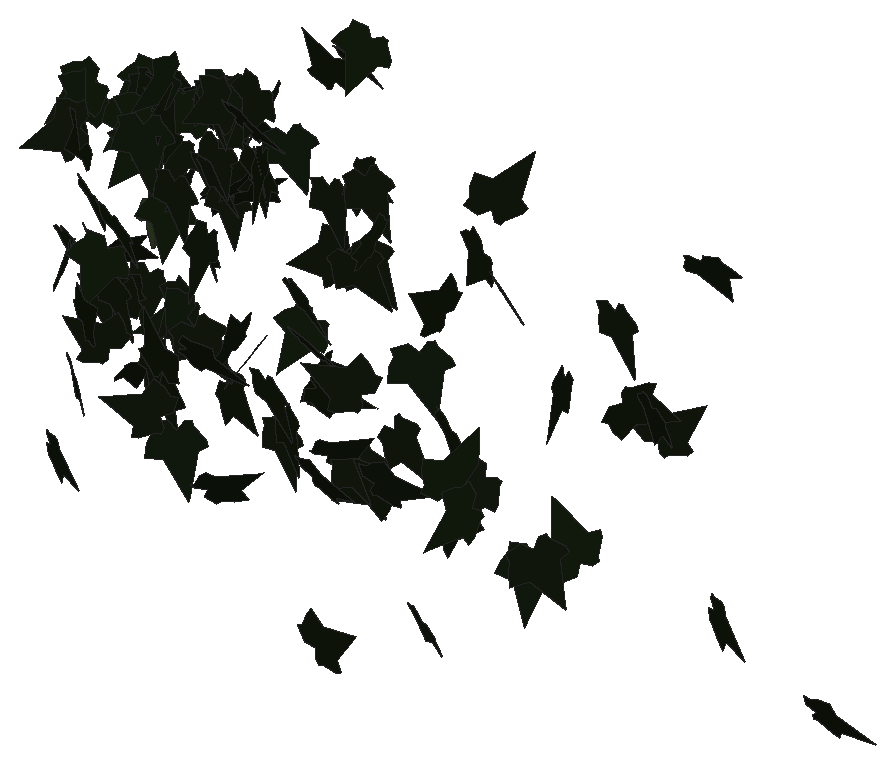
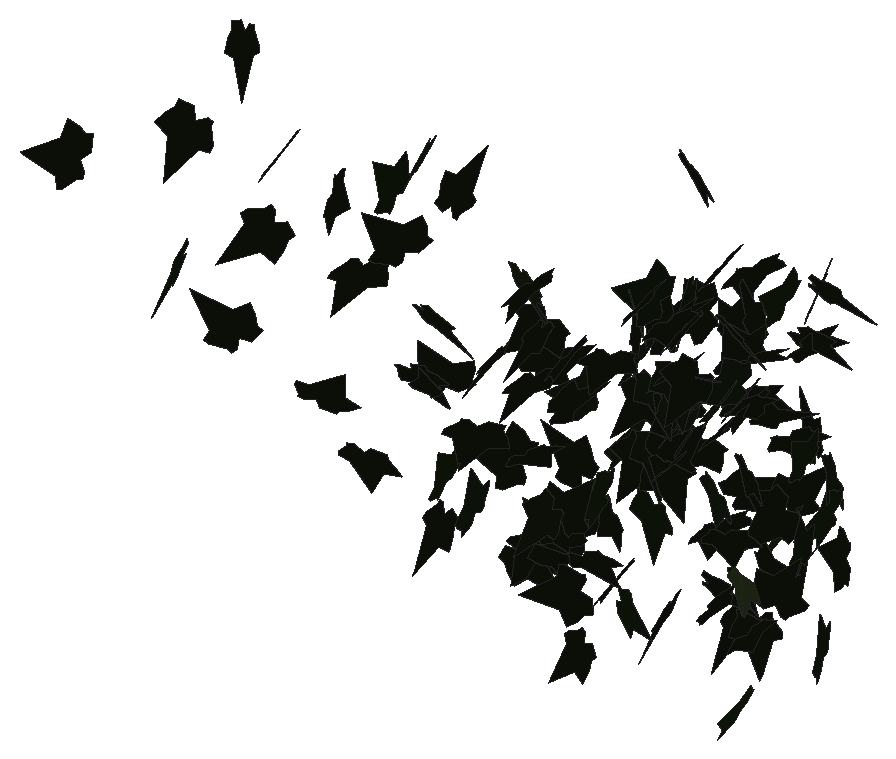
# SketchUp Ruby script. Lengths in inches.
U = 1.inch
M = Sketchup.active_model
def pt(a) = Geom::Point3d.new(a.map { |v| v * U })
def face(e, loops, mat)
  f = e.add_face(loops[0].map { |a| pt(a) })
  loops[1..].each { |l| e.add_face(l.map { |a| pt(a) }).erase! }
  f.material = f.back_material = mat if mat
  f
end
# faces: each face lists its corners as indices into pts; further lists are holes
def faces(e, pts, list, mat = nil) = list.each { |f| face(e, (f[0].is_a?(Array) ? f : [f]).map { |l| l.map { |i| pts[i] } }, mat) }
# xy, xz, yz: faces in a plane at the given z, y or x. An outline is a flat list of corners, or four numbers for a rectangle; further outlines are holes
def ring(l) = l.size == 4 ? [[l[0], l[1]], [l[2], l[1]], [l[2], l[3]], [l[0], l[3]]] : l.each_slice(2).to_a
def flat(e, list, mat, &to3) = list.each { |f| face(e, (f[0].is_a?(Array) ? f : [f]).map { |l| ring(l).map { |u, v| to3.(u, v) } }, mat) }
def xy(e, z, list, mat = nil) = flat(e, list, mat) { |x, y| [x, y, z] }
def xz(e, y, list, mat = nil) = flat(e, list, mat) { |x, z| [x, y, z] }
def yz(e, x, list, mat = nil) = flat(e, list, mat) { |y, z| [x, y, z] }
def lines(e, pts, list) = list.each { |a, b| e.add_line(pt(pts[a]), pt(pts[b])) }
# prism: a flat outline (further loops are holes) pulled along v
def prism(e, loops, v, mat = nil)
  f = face(e, loops, mat); d = Geom::Vector3d.new(v.map { |x| x * U })
  f.pushpull(f.normal.samedirection?(d) ? d.length : -d.length)
end
def box(e, o, s, mat = nil) = prism(e, [[o, [o[0] + s[0], o[1], o[2]], [o[0] + s[0], o[1] + s[1], o[2]], [o[0], o[1] + s[1], o[2]]]], [0, 0, s[2]], mat)
def at(x, y, z, deg = 0) = Geom::Transformation.translation(pt([x, y, z])) * Geom::Transformation.rotation(ORIGIN, Z_AXIS, deg.degrees)
def axes(o, x, y, z) = Geom::Transformation.new([*x, 0, *y, 0, *z, 0, *pt(o).to_a, 1])
def part(name) = M.definitions.add(name)
# library, detail: a bought-in or finely detailed component or shape, given as its bounding box
def library(name, o, s) = part(name).tap { |d| box(d.entities, o, s) }
def detail(e, o, s) = box(e.add_group.entities, o, s)
def put(e, d, t, mat = nil) = e.add_instance(d, t).tap { |i| i.material = mat if mat }
def group(e, t, mat = nil) = e.add_group.tap { |g| g.transformation = t; g.material = mat if mat }.entities
root = M.entities
M.materials.add("efeu1").color = [18, 25, 13]
M.materials.add("efeu2").color = [43, 57, 29]
c1 = part("ivyleaf_9")
p = [[1.54,2.16,1.25],[1.36,2.04,1.19],[-0.21,0.99,0.68],[-0.71,1.11,0.82],[-0.85,0.86,0.67],[-0.8,0.17,0.21],
  [-0.9,-0.01,0.1],[-0.67,-0.16,-0.02],[-0.08,-0.08,-0.05],[-0.03,-0.6,-0.4],[0.65,-0.88,-0.66],[0.83,-0.6,-0.49],
  [1.29,-0.42,-0.43],[1.8125,-0.07,-0.26],[1.21,0.44,0.15]]
faces(c1.entities,p,[[0,1,2,3,4,5,6,7,8,9,10,11,12,13,14]],"efeu1")
c2 = part("ivyleaf_10")
p = [[0,0.5,-0.03],[-0.0625,2.02,-0.43],[-0.19,2.01,-0.46],[-0.54,1.05,-0.29],[-0.52,0.625,-0.18],[-0.83,0.76,-0.28],
  [-1.16,0.64,-0.33],[-1.15,0.33,-0.24],[-0.77,-0.39,0.02],[-0.3,-0.51,0.16],[0.04,-0.48,0.23],[-0.02,2.01,-0.4375],
  [-0.06,2.01,-0.43],[0.04,-0.49,0.23],[0.67,-0.49,0.14],[1.38,0.36,-0.2],[1.375,0.51,-0.24],[0.81,0.65,-0.19],
  [0.62,0.59,-0.15],[0.6,1.09,-0.28],[0.5,1.23,-0.31]]
faces(c2.entities,p,[[0,1,2,3,4,5,6,7,8,9,10],[11,12,0,13,14,15,16,17,18,19,20]],"efeu2")
put(root,c1,axes([640.31,116.39,317.35],[1.16846,-0.88159,0.07129],[0.0667,-0.02996,-1.46364],[0.88195,1.17025,0.01624]))
put(root,c2,axes([640.9,124.67,315.8],[1.22207,-0.2873,0.16471],[0.19934,0.13529,-1.24301],[0.26445,1.22568,0.17581]))
put(root,c1,axes([641.4,136.23,319.18],[-0.91834,0.42729,-0.85127],[0.67528,-0.54188,-1.00047],[-0.67174,-1.12888,0.15803]))
put(root,c1,axes([640.67,119,315.09],[-0.02679,-0.37717,1.31538],[0.43757,-1.24892,-0.3492],[1.29654,0.41371,0.14503]))
put(root,c1,axes([641.8,120.08,312.01],[0.79627,-0.16263,1.10794],[-1.07914,0.25165,0.8125],[-0.29908,-1.34099,0.01811]))
put(root,c1,axes([641.22,123.75,311.48],[-0.09051,-1.27467,0.05842],[-0.03626,-0.05597,-1.27747],[1.27549,-0.09204,-0.03217]))
put(root,c1,axes([640.7,116.8125,307.07],[0.74096,-0.60878,-1.0482],[1.0596,-0.27136,0.90663],[-0.58871,-1.25464,0.31252]))
put(root,c1,axes([641.52,123.4375,323.16],[-0.67849,-0.09135,-1.09196],[1.09327,0.03031,-0.68184],[0.07401,-1.28522,0.06154]))
put(root,c1,axes([643.01,120.47,325.32],[-0.81227,0.08622,1.0327],[-1.00974,-0.36095,-0.76408],[0.23307,-1.26331,0.28879]))
put(root,c1,axes([642.73,116.17,329.4],[-1.35533,-0.27286,0.18589],[-0.17869,-0.05418,-1.38241],[0.27763,-1.36694,0.01768]))
put(root,c1,axes([641.59,117.83,313.6875],[0.61437,-1.24201,-0.09434],[-0.03171,0.08956,-1.3856],[1.24518,0.61508,0.01126]))
put(root,c1,axes([642.71,116.11,328.61],[-0.69237,-0.92516,0.77717],[-0.40045,-0.6694,-1.15362],[1.13998,-0.79705,0.06677]))
put(root,c1,axes([643.08,112.52,317.27],[-0.08249,0.66584,1.14036],[-0.08995,1.13709,-0.67044],[-1.31745,-0.11932,-0.02563]))
put(root,c1,axes([642.71,122.59,327.22],[-0.73308,-1.09231,0.05257],[0.08551,-0.12035,-1.30825],[1.09023,-0.72504,0.13796]))
put(root,c1,axes([642.05,116.9,320.68],[0.35585,-0.86092,0.90075],[0.43721,-0.79093,-0.92868],[1.16678,0.55894,0.07327]))
put(root,c1,axes([644.05,118.01,312.32],[-0.11258,0.1104,1.3975],[-0.92093,1.05121,-0.15723],[-1.05692,-0.92771,-0.01186]))
put(root,c1,axes([642.74,121.86,326.74],[0.37173,-1.3592,-0.17061],[-0.02655,0.1696,-1.40899],[1.36961,0.37219,0.01899]))
put(root,c1,axes([643.38,123.22,317.7],[-0.80166,-0.87771,-0.50482],[0.34134,0.37192,-1.18872],[0.95326,-0.87131,0.00112]))
put(root,c1,axes([642.87,122.73,304.78],[0.64586,-1.21892,0.28644],[0.15296,-0.24308,-1.3793],[1.24274,0.6634,0.02091]))
put(root,c1,axes([643.11,121.95,327.26],[0.44784,-1.22621,0.06593],[0.02248,-0.06198,-1.30544],[1.22778,0.44841,-0.00014]))
put(root,c1,axes([644.16,120.07,326.11],[-0.9206,-0.80956,0.49178],[-0.3784,-0.31436,-1.22586],[0.86836,-0.99526,-0.01283]))
put(root,c1,axes([643.47,117.37,316.88],[0.79356,0.92156,0.60672],[0.39451,0.46094,-1.21614],[-1.03041,0.88621,0.00163]))
put(root,c1,axes([644.75,118.34,308.8125],[0.09794,1.27164,-0.20626],[-0.02176,-0.20519,-1.27539],[-1.28807,0.10015,0.00587]))
put(root,c1,axes([643.85,116.56,315.11],[0.72763,-1.21166,0.00874],[0.00123,-0.00945,-1.41335],[1.21169,0.72762,-0.00381]))
put(root,c1,axes([645.14,121.97,319.52],[-0.10194,0.85981,0.97278],[-0.25922,0.94265,-0.86035],[-1.27216,-0.26097,0.09735]))
put(root,c1,axes([644.01,122.95,327.125],[0.66325,-1.12809,0.03312],[0.03442,-0.01818,-1.30846],[1.12805,0.66382,0.02045]))
put(root,c1,axes([645.72,110.84,329.53],[-1.3449,0.24778,0.53086],[-0.534,0.02819,-1.36602],[-0.24094,-1.4456,0.06436]))
put(root,c1,axes([643.82,121.43,327.7],[1.20649,-0.38811,0.45328],[0.51424,0.1575,-1.23388],[0.30275,1.27917,0.28945]))
put(root,c1,axes([645.15,122.68,311.53],[-0.32753,-0.97207,0.78046],[-0.21849,-0.74969,-1.02545],[1.22732,-0.39288,0.02572]))
put(root,c1,axes([646.7,120.57,311.79],[-1.22912,0.27794,0.5582],[-0.54049,0.14045,-1.26005],[-0.31098,-1.34261,-0.01626]))
put(root,c1,axes([645.55,121.46,323.65],[-0.14679,-1.24372,0.49099],[0.08462,-0.50159,-1.24527],[1.33444,-0.10501,0.13297]))
put(root,c1,axes([646.04,113.36,319.58],[-0.86186,-1.09961,-0.07568],[0.04896,0.05778,-1.39712],[1.10112,-0.86325,0.00288]))
put(root,c1,axes([645.82,111.5,328.39],[-0.20924,-0.37855,1.33222],[-0.0523,-1.34422,-0.39017],[1.38397,-0.10803,0.18667]))
put(root,c1,axes([646.9,118.95,330.04],[-1.3121,0.36922,-0.01084],[0.01033,-0.0033,-1.36306],[-0.36924,-1.31214,0.00038]))
put(root,c1,axes([647.11,135.22,322.92],[0.60569,-0.32306,1.15179],[-0.98669,0.59501,0.68576],[-0.67634,-1.15735,0.03105]))
put(root,c1,axes([647.24,121.45,326.78],[-1.21624,-0.23202,0.40606],[-0.31179,-0.441,-1.18586],[0.34857,-1.20401,0.3561]))
put(root,c1,axes([646.56,122.37,327.83],[0.75717,1.03684,0.2149],[0.14689,0.15879,-1.28364],[-1.04864,0.77089,-0.02464]))
put(root,c1,axes([647.3,111.94,313.67],[0.23699,0.12332,1.3102],[-1.23837,-0.42955,0.26443],[0.44527,-1.26027,0.03808]))
put(root,c1,axes([646.87,116.4375,326.38],[-0.89832,-0.97027,0.43051],[0.00478,-0.56767,-1.26943],[1.06148,-0.81857,0.37005]))
put(root,c1,axes([646.62,117.75,310.75],[-0.82029,-0.06383,-1.01081],[1.0089,0.06287,-0.82271],[0.08906,-1.30025,0.00984]))
put(root,c1,axes([647.11,117.35,307.86],[0.13524,-0.16457,-1.37499],[-0.86787,1.06649,-0.21301],[1.07911,0.87835,0.00101]))
put(root,c1,axes([647.05,136.6,324.07],[1.26694,0.10204,-0.21876],[-0.22709,0.10754,-1.26501],[-0.08184,1.28118,0.1236]))
put(root,c1,axes([646.43,107.39,308.03],[0.38473,-0.0408,-1.35161],[1.35157,0.05563,0.38304],[0.04236,-1.4042,0.05445]))
put(root,c1,axes([647.55,116.49,326.08],[-0.5221,-0.67272,1.24259],[0.86778,0.8928,0.84796],[-1.11514,1.00972,0.07809]))
put(root,c1,axes([648.54,122.93,320.94],[0.03629,1.18323,-0.56362],[-0.23016,-0.54932,-1.16802],[-1.29024,0.13127,0.1925]))
put(root,c1,axes([647.37,109.43,316.66],[-0.16548,0.14937,1.40214],[0.56376,-1.28701,0.20364],[1.29247,0.5805,0.09069]))
put(root,c1,axes([648.54,121.78,327],[0.05574,1.30094,-0.13778],[-0.15281,-0.13049,-1.2939],[-1.29926,0.07116,0.14627]))
put(root,c1,axes([648.75,122.85,320.95],[0.3879,0.03935,1.25108],[-1.24571,-0.11584,0.38988],[0.1223,-1.3047,0.00312]))
put(root,c1,axes([647.85,122.53,323.96],[0.36205,-1.24979,0.15719],[0.04594,-0.15035,-1.30118],[1.2588,0.36495,0.00227]))
put(root,c1,axes([647.97,121.34,323.08],[0.99655,-0.88618,-0.14908],[-0.10775,0.10317,-1.33357],[0.89215,1.00235,0.00546]))
put(root,c1,axes([649.47,122.89,326.49],[-0.2904,1.26792,-0.1074],[-0.13729,-0.14074,-1.29028],[-1.26503,-0.27579,0.16468]))
put(root,c1,axes([648.49,122.87,320.58],[0.15665,-1.29976,0.00646],[0.00508,-0.00589,-1.30916],[1.29977,0.15667,0.00434]))
put(root,c1,axes([648.34,113.95,326.94],[-0.22789,0.30578,1.36223],[0.65593,-1.19499,0.37797],[1.23245,0.69254,0.05072]))
put(root,c1,axes([649.49,122.7,325.93],[-0.09811,-1.2735,-0.30939],[-0.02233,-0.30858,1.27728],[-1.31036,0.10061,0.00139]))
put(root,c1,axes([649.65,122.71,321.91],[-0.13659,1.30686,-0.01214],[0.00021,-0.01218,-1.31397],[-1.30691,-0.13659,0.00106]))
put(root,c1,axes([649.29,120.1875,329.32],[0.37396,-1.26073,-0.04138],[-0.00314,0.04223,-1.31499],[1.26141,0.37387,0.00899]))
put(root,c1,axes([649.52,123.57,326.01],[1.29201,0.06514,-0.12699],[-0.12659,-0.01104,-1.29364],[-0.06591,1.29818,-0.00462]))
put(root,c1,axes([649.94,135.31,326.61],[-0.70895,-1.14555,0.14185],[0.08499,-0.21782,-1.3343],[1.15117,-0.68941,0.18587]))
put(root,c1,axes([649.75,112.61,330.24],[-0.1322,-1.43289,-0.42131],[0.06234,0.4173,-1.4388],[1.49225,-0.14437,0.02278]))
put(root,c1,axes([650.19,122.91,321.26],[0.68123,1.08107,0.28056],[0.09356,0.27224,-1.27618],[-1.11295,0.6846,0.06445]))
put(root,c1,axes([649.98,120.85,329.89],[-0.21578,-1.33295,-0.20263],[0.02964,0.20047,-1.3503],[1.34794,-0.21779,-0.00274]))
put(root,c1,axes([650.6,119.81,329.17],[-0.59004,-0.63206,1.05251],[-0.368,-1.023,-0.82065],[1.17126,-0.63983,0.27237]))
put(root,c1,axes([650.71,120.01,308.45],[0.80155,-0.81377,-0.91631],[-0.62803,0.66743,-1.14212],[1.05234,1.01816,0.01632]))
put(root,c1,axes([650.57,108.4,325.67],[0.67427,-1.06692,0.67998],[0.4379,-0.52609,-1.25968],[1.18698,0.80015,0.07845]))
put(root,c1,axes([652.97,109.98,311.48],[-0.31163,-0.05531,1.32072],[-1.29845,-0.24154,-0.31649],[0.24778,-1.33532,0.00254]))
put(root,c1,axes([652.52,120.85,330.14],[-0.13101,-1.18829,0.66611],[0.01001,-0.67,-1.19327],[1.36221,-0.10936,0.07283]))
put(root,c1,axes([653.15,125.72,307.33],[-0.12966,0.40737,-1.26995],[-0.71006,1.05899,0.41219],[1.12896,0.71284,0.1134]))
put(root,c1,axes([653.4,111.36,309.75],[-0.08109,-1.4151,-0.50641],[0.09499,0.50131,-1.41605],[1.49998,-0.10825,0.0623]))
put(root,c1,axes([654.26,123.93,312.57],[-1.18762,-0.62225,-0.08711],[0.0899,0.01607,-1.34048],[0.62186,-1.1907,0.02743]))
put(root,c1,axes([653.25,119.92,325.5],[0.35868,-1.21953,0.74235],[0.24621,-0.70112,-1.27075],[1.40632,0.43379,0.03314]))
put(root,c1,axes([652.89,118.3125,329.43],[0.89767,-0.69292,0.9461],[0.83488,-0.4591,-1.12838],[0.82354,1.22071,0.11266]))
put(root,c1,axes([654.64,116.61,312.87],[-0.22092,1.30626,0.52084],[-0.0807,0.51458,-1.3248],[-1.40395,-0.23512,-0.00581]))
put(root,c1,axes([653.71,122.24,326.65],[-0.3059,-0.93967,-0.88934],[0.31568,0.83203,-0.9877],[1.25469,-0.43843,0.03168]))
put(root,c1,axes([653.55,113.15,316.56],[-0.32512,-0.49084,-1.27348],[0.75185,1.02815,-0.58822],[1.13904,-0.81876,0.02478]))
put(root,c1,axes([653.73,110.79,328.28],[0.35656,-1.36006,0.11868],[0.05007,-0.10955,-1.40587],[1.36431,0.35947,0.02058]))
put(root,c1,axes([655.04,117.6875,326.84],[0.60001,-0.09941,-1.27835],[-1.24989,0.26958,-0.60761],[0.2861,1.38619,0.02648]))
put(root,c1,axes([654.5625,121.82,316.125],[1.17241,-0.86353,0.02651],[0.02112,-0.01603,-1.4561],[0.86368,1.1726,-0.00038]))
put(root,c1,axes([655.21,117.75,327.59],[-0.77802,0.08206,-1.19661],[1.17031,-0.26042,-0.77878],[-0.26267,-1.40334,0.07455]))
put(root,c1,axes([656.71,110.18,325.26],[0.7218,-0.04962,-1.16794],[-1.10407,0.42215,-0.70026],[0.38416,1.30647,0.18191]))
put(root,c1,axes([656.2,118.48,307.89],[0.48187,-1.31411,-0.02725],[-0.02318,0.02052,-1.39959],[1.31419,0.4822,-0.0147]))
put(root,c1,axes([655.96,122.63,308.96],[0.34443,0.34846,-1.27601],[0.84134,0.95973,0.48919],[1.02067,-0.9087,0.02736]))
put(root,c1,axes([657.63,104.49,318.99],[0.84904,-0.45567,1.0884],[-0.68129,0.90546,0.91054],[-0.96337,-1.04193,0.3153]))
put(root,c1,axes([657.95,121.25,324.81],[0.39738,-1.31613,-0.09347],[-0.03667,0.08657,-1.37477],[1.31893,0.39894,-0.01006]))
put(root,c1,axes([658.93,120.85,320.37],[-0.38823,-0.39136,1.26453],[-0.83628,-0.94899,-0.55046],[1.02609,-0.92152,0.02982]))
put(root,c1,axes([658.6,115.92,310.78],[-0.46309,-0.00804,-1.29447],[1.28749,0.13998,-0.46146],[0.1345,-1.36766,-0.03962]))
put(root,c1,axes([659.84,121.66,326.16],[0.50796,-0.34775,-1.19551],[-0.61694,1.05121,-0.56791],[1.08146,0.76303,0.23755]))
put(root,c1,axes([659.24,113.24,314.59],[0.77259,-1.23284,0.36713],[0.23775,-0.28402,-1.4541],[1.26418,0.80686,0.0491]))
put(root,c1,axes([660.11,108.58,319.5625],[0.32115,0.79492,1.08944],[-0.42334,-1.00387,0.85728],[1.28045,-0.53128,0.01019]))
put(root,c1,axes([659.45,105.22,320.55],[1.30617,-0.15942,0.65079],[0.64357,-0.09825,-1.31575],[0.18645,1.45601,-0.01753]))
put(root,c1,axes([661.43,104.3,329.91],[-1.15146,-0.0345,-0.92471],[0.92529,-0.06046,-1.14992],[-0.01099,-1.47557,0.06874]))
put(root,c1,axes([661.38,120.45,321.6],[0.32239,-1.05749,-0.93526],[-0.07943,0.94423,-1.09502],[1.4095,0.29508,0.15221]))
put(root,c1,axes([661.07,117.38,308.19],[1.14328,0.76944,-0.3911],[0.32573,0.21648,1.37809],[0.79931,-1.18877,-0.00219]))
put(root,c1,axes([661.38,114.32,317.91],[1.02214,-0.71119,0.69823],[0.68225,-0.22979,-1.23281],[0.72653,1.21634,0.17535]))
put(root,c1,axes([661.71,104.45,311.59],[1.03562,0.92054,-0.5268],[0.39813,0.34504,1.38559],[0.98306,-1.10949,-0.00619]))
put(root,c1,axes([661.625,115.11,307.77],[0.58866,-0.67747,1.19795],[0.9863,-0.70102,-0.8811],[0.95982,1.13586,0.17071]))
put(root,c1,axes([662.25,119.59,327.73],[0.38629,-1.30055,-0.54488],[-0.05303,0.55115,-1.35313],[1.40908,0.37728,0.09845]))
put(root,c1,axes([662.56,118.24,308],[-0.50812,-0.56858,-1.23636],[0.7633,0.97351,-0.7614],[1.12661,-0.91601,-0.04176]))
put(root,c1,axes([664.25,118.22,306.99],[0.052,0.08608,-1.43616],[-1.15328,-0.85671,-0.09311],[-0.86018,1.15382,0.03801]))
put(root,c1,axes([663.27,116.89,323.625],[-0.33998,-0.2818,-1.39283],[0.96045,1.00994,-0.43877],[1.04734,-1.01763,-0.04976]))
put(root,c1,axes([665.51,116.24,325.74],[-0.82032,1.07741,0.37079],[-0.23543,0.28676,-1.35409],[-1.11484,-0.85334,0.01312]))
put(root,c1,axes([667.07,112.75,316.86],[-0.15959,0.12087,1.418],[-1.41179,-0.19332,-0.14241],[0.1794,-1.41379,0.1407]))
put(root,c1,axes([666.22,120.09,316.11],[-0.51131,-0.98332,-0.98037],[0.45267,0.86961,-1.10831],[1.31268,-0.68289,0.00032]))
put(root,c1,axes([667.9,113.66,310.14],[0.74671,-0.22488,1.26706],[1.21813,-0.34884,-0.77978],[0.41494,1.42875,0.00904]))
put(root,c1,axes([668.82,120.01,311.4375],[0.29107,-0.96746,1.08973],[0.39136,-1.01853,-1.00878],[1.40368,0.48459,0.05529]))
put(root,c1,axes([670.95,117.67,306.93],[0.06256,-0.08833,-1.49007],[-0.92498,1.16823,-0.10808],[1.17155,0.92707,-0.00577]))
put(root,c1,axes([671.1,121.42,328.03],[-0.54006,-0.1683,1.40716],[1.31394,0.50478,0.56465],[-0.53102,1.42019,-0.03394]))
put(root,c1,axes([671.3125,111.34,316.14],[0.80899,-1.01172,-0.7666],[-0.27744,0.74614,-1.2775],[1.23866,0.82789,0.21454]))
put(root,c1,axes([671.14,103.47,303.88],[0.00715,0.02042,1.50665],[1.14935,-0.97437,0.00775],[0.97438,1.14919,-0.0202]))
put(root,c1,axes([673.81,110.85,303.35],[0.99569,-0.39264,-0.88837],[0.81766,-0.3478,1.07016],[-0.52421,-1.28827,-0.01816]))
put(root,c1,axes([674.81,111.74,325.9],[0.18777,0.19372,1.43585],[-0.86985,-1.14281,0.26794],[1.15868,-0.88933,-0.03154]))
put(root,c1,axes([675.01,112.3,312.8],[-0.93545,-0.22029,1.16347],[1.13776,0.24373,0.96092],[-0.32818,1.47287,0.015]))
put(root,c1,axes([675.64,114.61,329.21],[-0.0838,-0.86519,1.12515],[0.08172,-1.12818,-0.86143],[1.41698,0.01389,0.11622]))
put(root,c1,axes([676.75,113.4,313.65],[-1.34792,-0.42922,-0.17601],[0.16953,0.0477,-1.4146],[0.43182,-1.35853,0.00594]))
put(root,c1,axes([677.26,114.65,327.02],[0.43082,-0.81644,1.17668],[0.6676,-0.97262,-0.91928],[1.26707,0.79006,0.08427]))
put(root,c1,axes([679.61,108.4,314.7],[-1.47357,0.09058,-0.02],[0.01996,-0.00121,-1.47635],[-0.09058,-1.47371,-0.00001]))
put(root,c1,axes([678.99,115.52,307.75],[-1.05445,-0.71823,-0.7846],[0.67311,0.40489,-1.27526],[0.82364,-1.25041,0.03773]))
put(root,c1,axes([683.58,114.51,309.73],[-1.44276,-0.45103,-0.0833],[-0.06604,-0.0678,1.51095],[-0.45388,1.44358,0.04494]))
put(root,c1,axes([683.91,112.59,323.67],[-0.16269,0.16582,-1.43387],[1.14596,-0.86252,-0.22976],[-0.87764,-1.15695,-0.03422]))
put(root,c1,axes([685.43,116,327.64],[0.63365,-1.35624,0.03576],[0.0026,-0.03825,-1.4969],[1.35671,0.63351,-0.01383]))
put(root,c1,axes([685.3125,120.66,316.44],[-0.32096,-0.00029,1.42032],[1.3924,-0.28736,0.31459],[0.28023,1.42749,0.06362]))
put(root,c1,axes([686.39,106.54,314.79],[-0.04955,-0.99216,-1.12416],[0.04594,1.12324,-0.99337],[1.49867,-0.06724,-0.00672]))
put(root,c1,axes([686.67,115.43,321.77],[0.02502,0.07779,-1.48039],[-0.04667,1.47991,0.07698],[1.4817,0.0453,0.02743]))
put(root,c1,axes([688.95,120.5,330.62],[1.30383,0.60112,-0.31814],[-0.28375,-0.14437,-1.43568],[-0.6181,1.3343,-0.01201]))
put(root,c1,axes([695.96,106.58,328.47],[0.90774,0.08746,-1.15386],[-1.15146,-0.07716,-0.9117],[-0.11475,1.46609,0.02085]))
put(root,c1,axes([698.2,110.22,312.9],[1.07241,-0.62296,-0.85036],[-0.71453,0.46226,-1.23976],[0.775,1.28821,0.03366]))
put(root,c1,axes([711.51,104.15,312.85],[1.04069,-0.46918,0.9956],[0.94433,-0.32316,-1.13939],[0.56533,1.4035,0.07047]))
